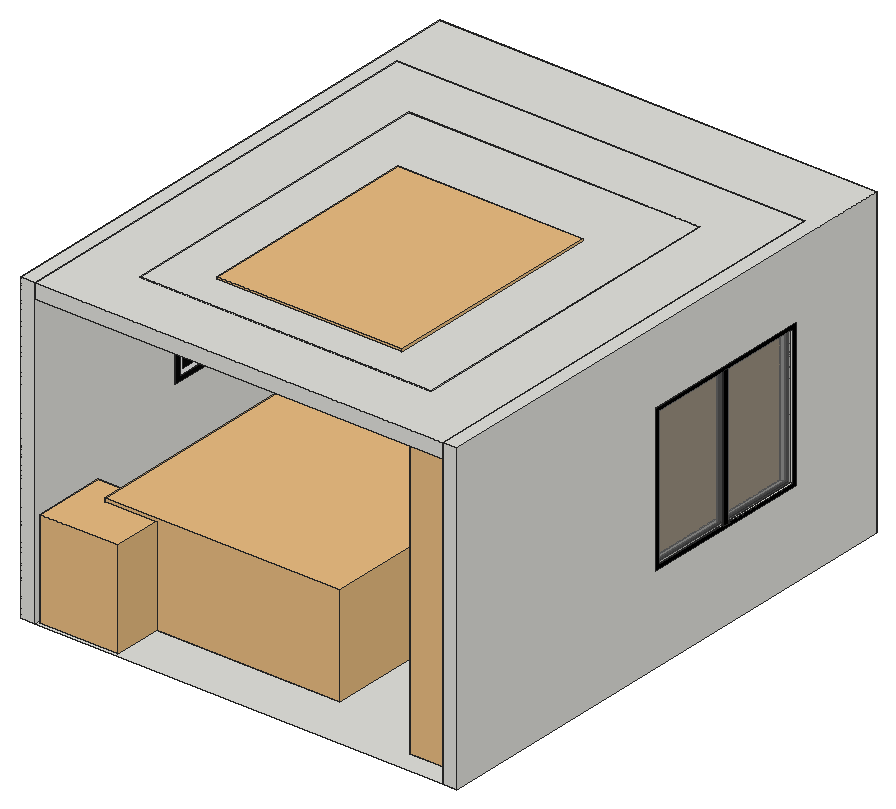
# SketchUp Ruby script. Lengths in inches.
U = 1.inch
M = Sketchup.active_model
def pt(a) = Geom::Point3d.new(a.map { |v| v * U })
def face(e, loops, mat)
  f = e.add_face(loops[0].map { |a| pt(a) })
  loops[1..].each { |l| e.add_face(l.map { |a| pt(a) }).erase! }
  f.material = f.back_material = mat if mat
  f
end
# faces: each face lists its corners as indices into pts; further lists are holes
def faces(e, pts, list, mat = nil) = list.each { |f| face(e, (f[0].is_a?(Array) ? f : [f]).map { |l| l.map { |i| pts[i] } }, mat) }
# xy, xz, yz: faces in a plane at the given z, y or x. An outline is a flat list of corners, or four numbers for a rectangle; further outlines are holes
def ring(l) = l.size == 4 ? [[l[0], l[1]], [l[2], l[1]], [l[2], l[3]], [l[0], l[3]]] : l.each_slice(2).to_a
def flat(e, list, mat, &to3) = list.each { |f| face(e, (f[0].is_a?(Array) ? f : [f]).map { |l| ring(l).map { |u, v| to3.(u, v) } }, mat) }
def xy(e, z, list, mat = nil) = flat(e, list, mat) { |x, y| [x, y, z] }
def xz(e, y, list, mat = nil) = flat(e, list, mat) { |x, z| [x, y, z] }
def yz(e, x, list, mat = nil) = flat(e, list, mat) { |y, z| [x, y, z] }
def lines(e, pts, list) = list.each { |a, b| e.add_line(pt(pts[a]), pt(pts[b])) }
# prism: a flat outline (further loops are holes) pulled along v
def prism(e, loops, v, mat = nil)
  f = face(e, loops, mat); d = Geom::Vector3d.new(v.map { |x| x * U })
  f.pushpull(f.normal.samedirection?(d) ? d.length : -d.length)
end
def box(e, o, s, mat = nil) = prism(e, [[o, [o[0] + s[0], o[1], o[2]], [o[0] + s[0], o[1] + s[1], o[2]], [o[0], o[1] + s[1], o[2]]]], [0, 0, s[2]], mat)
def at(x, y, z, deg = 0) = Geom::Transformation.translation(pt([x, y, z])) * Geom::Transformation.rotation(ORIGIN, Z_AXIS, deg.degrees)
def axes(o, x, y, z) = Geom::Transformation.new([*x, 0, *y, 0, *z, 0, *pt(o).to_a, 1])
def part(name) = M.definitions.add(name)
# library, detail: a bought-in or finely detailed component or shape, given as its bounding box
def library(name, o, s) = part(name).tap { |d| box(d.entities, o, s) }
def detail(e, o, s) = box(e.add_group.entities, o, s)
def put(e, d, t, mat = nil) = e.add_instance(d, t).tap { |i| i.material = mat if mat }
def group(e, t, mat = nil) = e.add_group.tap { |g| g.transformation = t; g.material = mat if mat }.entities
root = M.entities
M.materials.add("Plastic_Metalic_Black").color = [8, 8, 8]
M.materials.add("[Color M00]1").color = [254, 254, 254]
M.materials.add("[Color M00]2").color = [255, 255, 255]
M.materials.add("[Color_008]").color = [30, 30, 30]
M.materials.add("[Color_009]").color = [0, 0, 0]
M.materials.add("[Translucent_Glass_Gray]").color = [128, 128, 128]
M.materials["[Translucent_Glass_Gray]"].alpha = 0.5
c1 = library("Curtains and rod",[2.63,-1.46,0.02],[153.39,14.02,114.15])
c2 = part("Photos Gallery Wall")
g1 = group(c2.entities,at(0,0,0))
xy(g1,23.66,[[13.71,0.34,13.7,1.03,31.9375,1.12,31.94,0.43]],"Plastic_Metalic_Black")
xy(g1,24.66,[[14.71,0.34,30.94,0.42,30.9375,1.02,14.7,0.94]],"Plastic_Metalic_Black")
xy(g1,48.82,[[14.71,0.34,14.7,0.94,30.9375,1.02,30.94,0.42]],"Plastic_Metalic_Black")
xy(g1,49.82,[[13.71,0.34,31.94,0.43,31.9375,1.12,13.7,1.03]],"Plastic_Metalic_Black")
p = [[13.7,1.03,49.82],[13.7,1.03,23.66],[13.71,0.34,23.66],[13.71,0.34,49.82],[31.94,0.43,23.66],[31.94,0.43,49.82],
  [30.94,0.42,24.66],[14.71,0.34,24.66],[14.71,0.34,48.82],[30.94,0.42,48.82],[31.9375,1.12,23.66],[31.9375,1.12,49.82],
  [14.7,1.04,24.66],[30.9375,1.11,24.66],[30.9375,1.11,48.82],[14.7,1.04,48.82],[14.7,0.94,48.82],[14.7,0.94,24.66],
  [30.9375,1.02,24.66],[30.9375,1.02,48.82],[29.9375,1.02,47.82],[29.9375,1.02,25.66],[15.7,0.95,25.66],[15.7,0.95,47.82]]
faces(g1,p,[[0,1,2,3],[[4,5,3,2],[6,7,8,9]],[10,11,5,4],[[11,10,1,0],[12,13,14,15]],[16,8,7,17],[18,6,9,19],[21,20,23,22]],"Plastic_Metalic_Black")
faces(g1,p,[[[17,18,19,16],[20,21,22,23]]],"[Color M00]1")
lines(g1,p,[[14,19],[15,16],[12,17],[13,18]])
c3 = part("Photo+Frames+03")
put(c3.entities,c2,axes([128.61,79.32,-32.19],[1.3608,0,0],[0,1.3608,0],[0,0,1.3608]))
c4 = library("Platform bed",[0,0,0],[83.59,112.46,35.43])
c5 = library("SKT_Nearly Natural 5' Kentia Palm Silk Tree",[-23.18,-17.61,0],[47.48,43.95,59.125])
c6 = library("Round wall hanging",[0,0,0],[26.88,1.18,49.49])
c7 = library("ceiling fan",[0,0,0],[76.25,93.13,30.02])
c8 = part("Component\#1")
xy(c8.entities,0,[[4,0,5.04,0.14,6,0.54,6.83,1.17,7.46,2,7.86,2.96,8,4,7.86,5.04,7.46,6,6.83,6.83,6,7.46,5.04,7.86,4,8,2.96,7.86,2,7.46,1.17,6.83,0.54,6,0.14,5.04,0,4,0.14,2.96,0.54,2,1.17,1.17,2,0.54,2.96,0.14]],"[Color M00]2")
xy(root,0,[[0,0,6,0,6,186.5,102,186.5,102,210,174,210,174,0,180,0,180,216,0,216],[6,0,174,186.5]])
xy(root,1,[[102,186.5,174,210]])
xy(root,1.2,[[7.2,186,30.3,186.5],[30.7,186,53.8,186.5],[54.2,186,77.3,186.5],[77.7,186,100.8,186.5]])
xy(root,19.5,[[102,186.5,174,210]])
xy(root,20.5,[[102,186.5,174,210]])
xy(root,36,[[174,102,180,174]])
xy(root,39.5,[[102,186.5,174,210]])
xy(root,40.5,[[102,186.5,174,210]])
xy(root,59.5,[[102,186.5,174,210]])
xy(root,60.5,[[102,186.5,174,210]])
xy(root,79.5,[[102,186.5,174,210]])
xy(root,80.5,[[102,186.5,174,210]])
xy(root,88.9,[[7.2,186,30.3,186.5],[30.7,186,53.8,186.5],[54.2,186,77.3,186.5],[77.7,186,100.8,186.5]])
xy(root,91.1,[[7.2,186,30.3,186.5],[30.7,186,53.8,186.5],[54.2,186,77.3,186.5],[77.7,186,100.8,186.5]])
xy(root,96,[[174,102,180,174]])
xy(root,99.5,[[102,186.5,174,210]])
xy(root,100.5,[[102,186.5,137.5,186.68],[137.5,186.5,173,186.68]])
xy(root,100.7,[[102.2,186.5,137.3,186.68],[137.7,186.5,172.8,186.68]])
xy(root,118.8,[[7.2,186,30.3,186.5],[30.7,186,53.8,186.5],[54.2,186,77.3,186.5],[77.7,186,100.8,186.5],[102.2,186.5,137.3,186.68],
  [137.7,186.5,172.8,186.68]])
xy(root,119,[[102,186.5,137.5,186.68],[137.5,186.5,173,186.68]])
xy(root,126,[[0,0,6,0,6,186.5,174,186.5,174,0,180,0,180,216,0,216]])
xz(root,0,[[0,0,6,126],[174,0,180,126]])
xz(root,102,[[174,36,180,96]])
xz(root,174,[[174,36,180,96]])
xz(root,186,[[7.2,1.2,30.3,88.9],[30.7,1.2,53.8,88.9],[54.2,1.2,77.3,88.9],[77.7,1.2,100.8,88.9],[7.2,91.1,30.3,118.8],
  [30.7,91.1,53.8,118.8],[54.2,91.1,77.3,118.8],[77.7,91.1,100.8,118.8]])
xz(root,186.5,[[[6,0,102,0,102,119,173,119,173,100.5,174,100.5,174,126,6,126],[7,1,101,89.1],[7,90.9,101,119]],[102,0,174,1],[[7,1,101,89.1],[77.7,1.2,100.8,88.9],[54.2,1.2,77.3,88.9],[30.7,1.2,53.8,88.9],[7.2,1.2,30.3,88.9]],[102,19.5,174,20.5],[102,39.5,174,40.5],
  [102,59.5,174,60.5],[102,79.5,174,80.5],[[7,90.9,101,119],[77.7,91.1,100.8,118.8],[54.2,91.1,77.3,118.8],[7.2,91.1,30.3,118.8],[30.7,91.1,53.8,118.8]],[102,99.5,174,100.5],[102.2,100.7,137.3,118.8],
  [137.7,100.7,172.8,118.8]])
xz(root,186.68,[[[102,100.5,173,119],[102.2,100.7,137.3,118.8],[137.7,100.7,172.8,118.8]]])
xz(root,210,[[102,0,174,1],[102,1,174,19.5],[102,20.5,174,39.5],[102,40.5,174,59.5],[102,60.5,174,79.5],
  [102,80.5,174,99.5]])
xz(root,216,[[0,0,180,126]])
yz(root,0,[[0,0,216,126]])
yz(root,6,[[0,0,186.5,126]])
yz(root,7.2,[[186,1.2,186.5,88.9],[186,91.1,186.5,118.8]])
yz(root,30.3,[[186,1.2,186.5,88.9],[186,91.1,186.5,118.8]])
yz(root,30.7,[[186,1.2,186.5,88.9],[186,91.1,186.5,118.8]])
yz(root,53.8,[[186,1.2,186.5,88.9],[186,91.1,186.5,118.8]])
yz(root,54.2,[[186,1.2,186.5,88.9],[186,91.1,186.5,118.8]])
yz(root,77.3,[[186,1.2,186.5,88.9],[186,91.1,186.5,118.8]])
yz(root,77.7,[[186,1.2,186.5,88.9],[186,91.1,186.5,118.8]])
yz(root,100.8,[[186,1.2,186.5,88.9],[186,91.1,186.5,118.8]])
yz(root,102,[[186.5,0,210,1],[186.5,1,210,19.5],[186.5,20.5,210,39.5],[186.5,40.5,210,59.5],[186.5,60.5,210,79.5],
  [186.5,80.5,210,99.5],[186.5,100.5,186.68,119]])
yz(root,102.2,[[186.5,100.7,186.68,118.8]])
yz(root,137.3,[[186.5,100.7,186.68,118.8]])
yz(root,137.7,[[186.5,100.7,186.68,118.8]])
yz(root,172.8,[[186.5,100.7,186.68,118.8]])
yz(root,173,[[186.5,100.5,186.68,119]])
yz(root,174,[[[0,0,0,126,186.5,126,186.5,99.5,210,99.5,210,80.5,186.5,80.5,186.5,79.5,210,79.5,210,60.5,186.5,60.5,186.5,59.5,210,59.5,210,40.5,186.5,40.5,186.5,39.5,210,39.5,210,20.5,186.5,20.5,186.5,19.5,210,19.5,210,1,186.5,1,186.5,0],[102,36,174,96]],[186.5,0,210,1]])
yz(root,180,[[[0,0,216,126],[102,36,174,96]]])
p = [[367.529,-740.22,227.771],[367.527,-740.22,227.771],[367.527,-740.22,226.735],[367.529,-740.22,226.735]]
lines(root,p,[[0,1],[2,3]])
put(root,c1,axes([161.44,189.68,5.83],[0,-1.21,0],[1,0,0],[0,0,1]))
put(root,c3,axes([86.72,-141.84,57.34],[0,1.45,0],[-1,0,0],[0,0,1.28]))
put(root,c4,axes([114.59,152.01,0],[-1.16,0,0],[0,-1.16,0],[0,0,1.16]))
put(root,c5,axes([22.5,13.66,-0.26],[0.68,0,0],[0,0.68,0],[0,0,0.68]))
put(root,c6,axes([9.54,134.99,74.75],[0,0.58,0],[-3,0,0],[0,0,0.58]))
g2 = group(root,at(177.18,174,36))
xy(g2,0,[[0,-72,3.17,0]],"[Color_009]")
xy(g2,1.43,[[2.64,-70.29,3.17,-36.86],[2.64,-35.14,3.17,-1.71]])
xy(g2,1.43,[[0,-70.29,0.79,-36.86],[0,-35.14,0.79,-1.71]],"[Color_009]")
xy(g2,58.57,[[0,-70.29,0.79,-36.86],[0.79,-70.29,2.64,-36.86],[2.64,-70.29,3.17,-36.86],[0,-35.14,0.79,-1.71],[0.79,-35.14,2.64,-1.71],
  [2.64,-35.14,3.17,-1.71]])
xy(g2,60,[[0,-72,3.17,0]],"[Color_008]")
xz(g2,-72,[[0,0,3.17,60]],"[Color_009]")
xz(g2,-70.29,[[0,1.43,0.79,58.57],[2.64,1.43,3.17,58.57]],"[Color_009]")
xz(g2,-36.86,[[0,1.43,0.79,58.57],[2.64,1.43,3.17,58.57]])
xz(g2,-35.14,[[0,1.43,0.79,58.57],[2.64,1.43,3.17,58.57]],"[Color_009]")
xz(g2,-1.71,[[2.64,1.43,3.17,58.57]])
xz(g2,-1.71,[[0,1.43,0.79,58.57]],"[Color_009]")
xz(g2,0,[[0,0,3.17,60]],"[Color_009]")
yz(g2,0,[[[-72,0,0,60],[-35.14,1.43,-1.71,58.57],[-70.29,1.43,-36.86,58.57]]],"[Color_009]")
yz(g2,0.79,[[-70.29,1.43,-36.86,58.57],[-35.14,1.43,-1.71,58.57]],"[Translucent_Glass_Gray]")
yz(g2,2.64,[[-70.29,1.43,-36.86,58.57],[-35.14,1.43,-1.71,58.57]],"[Translucent_Glass_Gray]")
yz(g2,3.17,[[[-72,0,0,60],[-70.29,1.43,-1.71,58.57]],[-36.86,1.43,-35.14,58.57]],"[Color_009]")
g3 = group(root,at(6,0,96.74))
put(g3,c7,axes([44.16,38.71,8.7],[1,0,0],[0,1,0],[0,0,0.71]))
g4 = group(g3,at(0,0,23.26))
put(g4,c8,at(8.25,7.9375,0))
put(g4,c8,at(81.4375,172,0))
put(g4,c8,at(8.25,63.5625,0))
put(g4,c8,at(151.9375,7.9375,0),"[Color M00]2")
put(g4,c8,at(8.25,120,0))
put(g4,c8,at(151.9375,172.1875,0))
put(g4,c8,at(81.4375,7.9375,0))
put(g4,c8,at(151.9375,120,0))
put(g4,c8,at(8.25,172.1875,0))
put(g4,c8,at(151.9375,63.5625,0))
g5 = group(g4,at(0,0,6))
xy(g5,-6,[[[0,0,168,186.5],[24,24,144,162.5]]])
xy(g5,0,[[[0,0,168,186.5],[24,24,144,162.5]],[24,24,144,162.5]])
xz(g5,0,[[0,-6,168,0]])
xz(g5,24,[[24,-6,144,0]])
xz(g5,162.5,[[24,-6,144,0]])
xz(g5,186.5,[[0,-6,168,0]])
yz(g5,0,[[0,-6,186.5,0]])
yz(g5,24,[[24,-6,162.5,0]])
yz(g5,144,[[24,-6,162.5,0]])
yz(g5,168,[[0,-6,186.5,0]])
